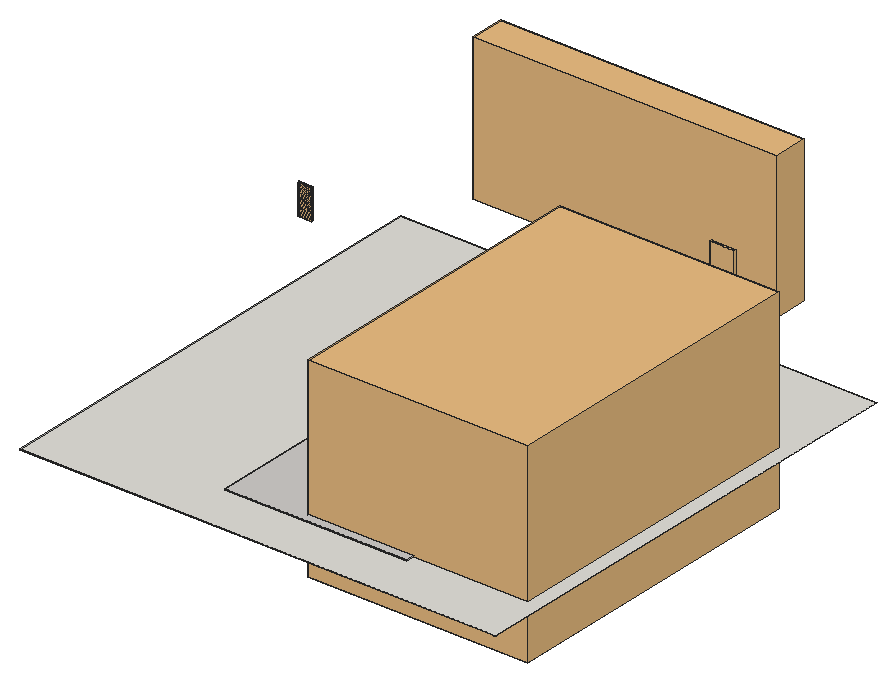
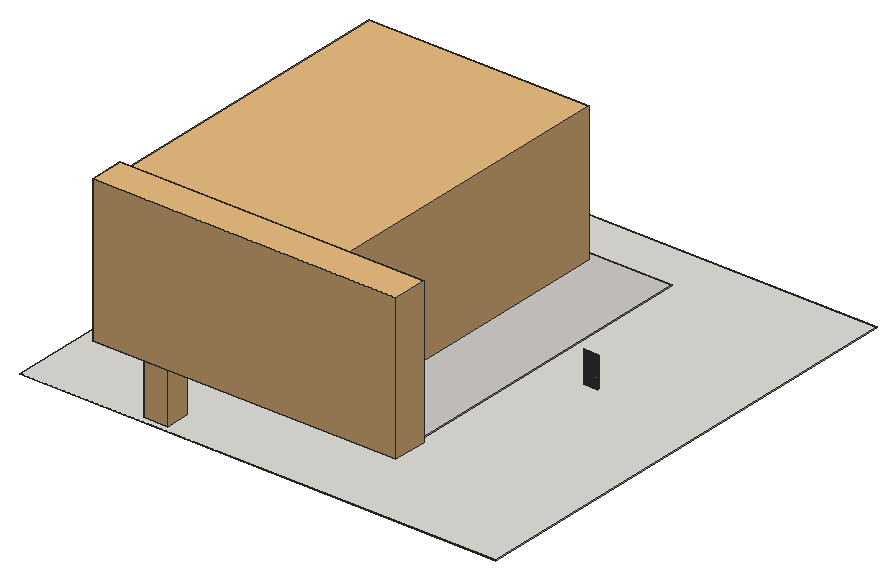
# SketchUp Ruby script. Lengths in inches.
U = 1.inch
M = Sketchup.active_model
def pt(a) = Geom::Point3d.new(a.map { |v| v * U })
def face(e, loops, mat)
  f = e.add_face(loops[0].map { |a| pt(a) })
  loops[1..].each { |l| e.add_face(l.map { |a| pt(a) }).erase! }
  f.material = f.back_material = mat if mat
  f
end
# faces: each face lists its corners as indices into pts; further lists are holes
def faces(e, pts, list, mat = nil) = list.each { |f| face(e, (f[0].is_a?(Array) ? f : [f]).map { |l| l.map { |i| pts[i] } }, mat) }
# xy, xz, yz: faces in a plane at the given z, y or x. An outline is a flat list of corners, or four numbers for a rectangle; further outlines are holes
def ring(l) = l.size == 4 ? [[l[0], l[1]], [l[2], l[1]], [l[2], l[3]], [l[0], l[3]]] : l.each_slice(2).to_a
def flat(e, list, mat, &to3) = list.each { |f| face(e, (f[0].is_a?(Array) ? f : [f]).map { |l| ring(l).map { |u, v| to3.(u, v) } }, mat) }
def xy(e, z, list, mat = nil) = flat(e, list, mat) { |x, y| [x, y, z] }
def xz(e, y, list, mat = nil) = flat(e, list, mat) { |x, z| [x, y, z] }
def yz(e, x, list, mat = nil) = flat(e, list, mat) { |y, z| [x, y, z] }
def lines(e, pts, list) = list.each { |a, b| e.add_line(pt(pts[a]), pt(pts[b])) }
# prism: a flat outline (further loops are holes) pulled along v
def prism(e, loops, v, mat = nil)
  f = face(e, loops, mat); d = Geom::Vector3d.new(v.map { |x| x * U })
  f.pushpull(f.normal.samedirection?(d) ? d.length : -d.length)
end
def box(e, o, s, mat = nil) = prism(e, [[o, [o[0] + s[0], o[1], o[2]], [o[0] + s[0], o[1] + s[1], o[2]], [o[0], o[1] + s[1], o[2]]]], [0, 0, s[2]], mat)
def at(x, y, z, deg = 0) = Geom::Transformation.translation(pt([x, y, z])) * Geom::Transformation.rotation(ORIGIN, Z_AXIS, deg.degrees)
def axes(o, x, y, z) = Geom::Transformation.new([*x, 0, *y, 0, *z, 0, *pt(o).to_a, 1])
def part(name) = M.definitions.add(name)
# library, detail: a bought-in or finely detailed component or shape, given as its bounding box
def library(name, o, s) = part(name).tap { |d| box(d.entities, o, s) }
def detail(e, o, s) = box(e.add_group.entities, o, s)
def put(e, d, t, mat = nil) = e.add_instance(d, t).tap { |i| i.material = mat if mat }
def group(e, t, mat = nil) = e.add_group.tap { |g| g.transformation = t; g.material = mat if mat }.entities
root = M.entities
M.materials.add("BED RUG").color = [207, 204, 201]
M.materials.add("[Marble Carrara Gold Floor Tile]").color = [225, 223, 217]
M.materials.add("green").color = [174, 139, 102]
c1 = part("3DGeom~106_Defintion")
p = [[13,-457.77,-202.36],[12.43,-457.8,-202.3125],[13.01,-486.125,-217.66],[13.55,-486.1,-217.7],[11.89,-399.92,-173.32],[11.84,-429.07,-187.52],
  [12.45,-429.04,-187.5625],[11.24,-399.94,-173.27],[10.74,-340.47,-146.51],[10.02,-340.5,-146.45],[10.64,-370.42,-159.59],[11.32,-370.39,-159.64],
  [9.74,-274.82,-123],[9.45,-308.6875,-134.19],[10.21,-308.66,-134.25],[8.94,-274.85,-122.9375],[8.71,-207.8125,-101.79],[7.83,-207.84,-101.72],
  [8.42,-240.67,-112.26],[9.26,-240.64,-112.32],[7.13,-153.09,-79.54],[7.1,-178.08,-90.92],[8.02,-178.05,-90.99],[6.18,-153.15,-79.48],
  [4,-118.48,-55.33],[4.82,-133.72,-67.51],[5.79,-133.63,-67.55],[3.02,-118.6,-55.3],[0.33,-95.6,-29.9375],[-0.7,-95.73,-29.92],
  [1.08,-106.39,-42.81],[2.09,-106.26,-42.82],[-1.44,-73.6,-2.8],[-2,-85.27,-16.55],[-0.96,-85.15,-16.59],[-2.51,-73.67,-2.71],
  [0.95,-49.78,26.84],[-1.83,-61.59,11.65],[-0.75,-61.55,11.52],[0.95,-49.78,26.84],[-0.16,-49.81,27.01],[5.32,-27.04,58.03],
  [2.02,-38.3,42.73],[3.14,-38.29,42.55],[5.32,-27.04,58.03],[4.18,-27.0625,58.2],[7.55,-5.16,85.82],[5.8,-16.06,72.8],
  [6.97,-16.01,72.65],[6.36,-5.25,85.91],[4.9,15.04,108.74],[3.7,14.85,108.73],[5.55,5,97.6],[6.74,5.15,97.57],
  [0,34.3,128.09],[-1.23,34.1,128.07],[1.28,24.49,118.99],[2.49,24.7,119.02],[-3.26,54.16,141.33],[-4.54,54.09,141.39],
  [-3.34,43.89,135.65],[-2.08,44.05,135.64],[1.2,113.2,138.8],[-0.38,104.875,137.27],[0.95,104.81,137.18],[-0.15,113.16,138.875],
  [0.07,95.73,138.14],[-2.47,86.16,140.63],[-1.16,86.02,140.55],[-1.25,95.85,138.22],[-2.41,75.83,143.01],[-3.7,75.9375,143.09],
  [-4.55,65.2,143.98],[-3.26,65.16,143.89],[-0.4,131.04,151.24],[-0.67,121.83,143.76],[0.69,121.94,143.73],[-1.77,130.9,151.24],
  [-3.3125,149.46,169.92],[-4.71,149.31,169.92],[-3.22,140.1,160.31],[-1.83,140.26,160.32],[-5.28,167.68,186.64],[-5.98,158.46,179.0625],
  [-4.5625,158.59,179.04],[-6.71,167.6,186.71],[-4.84,183.58,197.42],[-6.74,175.84,192.46],[-5.3,175.86,192.35],[-6.28,183.61,197.56],
  [-3.32,198.87,205.72],[-5.56,191.21,202.02],[-4.1,191.16,201.87],[-4.79,198.92,205.87],[-2.54,215.74,211.62],[-4.2,207,209.1],
  [-2.73,206.98,208.96],[-4.03,215.71,211.74],[-3.51,234.5625,213.875],[-4.36,225.09,213.4375],[-2.87,225.16,213.32],[-5.02,234.48,213.99],
  [-5.16,253.86,213.61],[-6.6875,253.77,213.74],[-5.84,243.98,213.93],[-4.32,244.07,213.8125],[-6.4,274.98,214.6],[-7.43,264.02,213.86],
  [-5.89,264.1,213.73],[-7.96,274.93,214.73],[-6.84,297.22,218.75],[-8.26,286.04,216.51],[-6.68,286.08,216.38],[-8.43,297.18,218.89],
  [-6.9375,322.55,224.28],[-8.52,309.11,221.61],[-6.91,309.14,221.48],[-8.56,322.52,224.42],[-6.99,356.56,229.06],[-8.59,338.11,227.04],
  [-6.95,338.125,226.9],[-8.65,356.54,229.2],[-7.09,400.64,232.43],[-8.73,377.54,230.99],[-7.05,377.56,230.84],[-8.81,400.63,232.57],
  [-7.16,453.07,235],[-8.875,425.8,233.96],[-7.13,425.81,233.8125],[-8.93,453.07,235.16],[-7.18,513.875,236.79],[-8.98,482.42,236.15],
  [-7.17,482.43,236],[-9.02,513.875,236.95]]
faces(c1.entities,p,[[0,1,2],[0,2,3],[4,5,6],[4,7,5],[8,9,10],[8,10,11],[12,13,14],[12,15,13],
  [16,17,18],[16,18,19],[20,21,22],[20,23,21],[24,25,26],[24,27,25],[28,29,30],[28,30,31],
  [32,33,34],[32,35,33],[36,37,38],[39,40,37],[41,42,43],[44,45,42],[46,47,48],[46,49,47],
  [50,51,52],[50,52,53],[54,55,56],[54,56,57],[58,59,60],[58,60,61],[62,63,64],[62,65,63],
  [66,67,68],[66,69,67],[70,71,72],[70,72,73],[74,75,76],[74,77,75],[78,79,80],[78,80,81],
  [82,83,84],[82,85,83],[86,87,88],[86,89,87],[90,91,92],[90,93,91],[94,95,96],[94,97,95],
  [98,99,100],[98,101,99],[102,103,104],[102,104,105],[106,107,108],[106,109,107],[110,111,112],[110,113,111],
  [114,115,116],[114,117,115],[118,119,120],[118,121,119],[122,123,124],[122,125,123],[126,127,128],[126,129,127],
  [130,131,132],[130,133,131]],"green")
c2 = part("3DGeom~107_Defintion")
p = [[13.6,-487.82,-218.47],[13.05,-487.84,-218.43],[13.63,-515.87,-234.39],[14.13,-515.85,-234.43],[12.5,-430.56,-188.23],[12.47,-459.41,-203.03],
  [13.05,-459.39,-203.07],[11.88,-430.58,-188.18],[11.36,-371.7,-160.2],[10.67,-371.73,-160.15],[11.28,-401.36,-173.89],[11.93,-401.33,-173.94],
  [10.25,-309.75,-134.72],[9.49,-309.78,-134.66],[10.06,-341.7,-146.97],[10.78,-341.67,-147.02],[9.29,-241.49,-112.72],[8.45,-241.52,-112.65],
  [8.97,-275.82,-123.37],[9.77,-275.8,-123.4375],[8.05,-178.67,-91.3125],[7.86,-208.57,-102.08],[8.74,-208.55,-102.15],[7.13,-178.71,-91.24],
  [5.81,-134.1,-67.79],[4.83,-134.1875,-67.74],[6.2,-153.69,-79.76],[7.16,-153.63,-79.82],[2.09,-106.64,-42.97],[1.09,-106.77,-42.96],
  [3.03,-119.01,-55.5],[4.02,-118.9,-55.53],[-0.96,-85.46,-16.65],[-2.01,-85.57,-16.6],[-0.7,-96.07,-30.02],[0.33,-95.9375,-30.04],
  [-0.75,-61.77,11.56],[-2.52,-73.93,-2.72],[-1.45,-73.86,-2.81],[-1.84,-61.81,11.7],[3.15,-38.42,42.7],[-0.16,-49.98,27.1],
  [0.95,-49.96,26.9375],[2.03,-38.4375,42.88],[6.99,-16.07,72.91],[4.19,-27.16,58.41],[5.34,-27.14,58.23],[5.82,-16.12,73.06],
  [6.77,5.17,97.91],[6.39,-5.26,86.21],[7.58,-5.17,86.12],[5.56,5.02,97.95],[2.5,24.78,119.4375],[1.28,24.58,119.41],
  [3.71,14.9,109.11],[4.92,15.09,109.12],[-2.09,44.21,136.12],[-3.35,44.05,136.13],[-1.23,34.22,128.52],[0,34.42,128.54],
  [0.96,105.18,137.67],[-1.25,96.19,138.71],[0.07,96.06,138.625],[-0.38,105.24,137.76],[0.7,122.37,144.24],[-0.15,113.56,139.37],
  [1.21,113.6,139.29],[-0.67,122.26,144.27],[-1.17,86.33,141.05],[-3.72,76.2,143.59],[-2.41,76.09,143.51],[-2.48,86.46,141.125],
  [-3.27,65.39,144.4],[-4.56,54.28,141.89],[-3.27,54.35,141.83],[-4.57,65.43,144.49],[-1.84,140.75,160.88],[-3.23,140.59,160.875],
  [-1.78,131.36,151.78],[-0.41,131.5,151.77],[-4.58,159.15,179.67],[-6,159.02,179.69],[-4.73,149.83,170.52],[-3.33,149.99,170.52],
  [-5.32,176.48,193.03],[-6.74,168.19,187.37],[-5.3,168.27,187.3],[-6.76,176.46,193.14],[-4.12,191.83,202.58],[-6.31,184.26,198.26],
  [-4.85,184.23,198.12],[-5.58,191.88,202.74],[-2.73,207.71,209.7],[-4.8,199.62,206.59],[-3.33,199.57,206.44],[-4.22,207.73,209.84],
  [-2.875,225.96,214.07],[-4.05,216.47,212.49],[-2.55,216.5,212.36],[-4.38,225.89,214.19],[-5.91,265.03,214.49],[-6.71,254.67,214.49],
  [-5.17,254.76,214.37],[-7.46,264.96,214.61],[-4.33,244.9375,214.57],[-5.86,244.84,214.6875],[-5.03,235.3,214.75],[-3.52,235.39,214.63],
  [-6.71,287.09,217.15],[-7.99,275.9,215.49],[-6.42,275.95,215.36],[-8.29,287.05,217.28],[-6.9375,310.23,222.26],[-8.46,298.23,219.66],
  [-6.87,298.27,219.53],[-8.55,310.2,222.39],[-6.97,339.32,227.7],[-8.59,323.66,225.21],[-6.96,323.68,225.07],[-8.62,339.3,227.84],
  [-7.07,378.89,231.66],[-8.68,357.8,230.01],[-7.02,357.82,229.87],[-8.76,378.88,231.8],[-7.16,427.3125,234.64],[-8.84,402.04,233.39],
  [-7.12,402.05,233.25],[-8.91,427.31,234.79],[-7.2,484.13,236.83],[-8.96,454.67,235.99],[-7.18,454.67,235.83],[-9.01,484.125,236.99]]
faces(c2.entities,p,[[0,1,2],[0,2,3],[4,5,6],[4,7,5],[8,9,10],[8,10,11],[12,13,14],[12,14,15],
  [16,17,18],[16,18,19],[20,21,22],[20,23,21],[24,25,26],[24,26,27],[28,29,30],[28,30,31],
  [32,33,34],[32,34,35],[36,37,38],[36,39,37],[40,41,42],[40,43,41],[44,45,46],[44,47,45],
  [48,49,50],[48,51,49],[52,53,54],[52,54,55],[56,57,58],[56,58,59],[60,61,62],[60,63,61],
  [64,65,66],[64,67,65],[68,69,70],[68,71,69],[72,73,74],[72,75,73],[76,77,78],[76,78,79],
  [80,81,82],[80,82,83],[84,85,86],[84,87,85],[88,89,90],[88,91,89],[92,93,94],[92,95,93],
  [96,97,98],[96,99,97],[100,101,102],[100,103,101],[104,105,106],[104,106,107],[108,109,110],[108,111,109],
  [112,113,114],[112,115,113],[116,117,118],[116,119,117],[120,121,122],[120,123,121],[124,125,126],[124,127,125],
  [128,129,130],[128,131,129]],"green")
c3 = library("3DGeom~108_Defintion",[-15.55,-485.98,-221.31],[30.67,1000,457.14])
c4 = library("3DGeom~109_Defintion",[-10.83,-486.12,-217.86],[24.87,1000,454.81])
c5 = library("3DGeom~110_Defintion",[-15.46,-515.69,-237.75],[31.06,1000,473.61])
c6 = library("3DGeom~111_Defintion",[-10.8,-515.86,-234.58],[25.39,1000,471.56])
c7 = library("3DGeom~112_Defintion",[-15.55,-486.02,-221.29],[30.67,1000,457.87])
c8 = library("3DGeom~113_Defintion",[-15.46,-515.73,-237.74],[31.06,1000,474.35])
c9 = part("3DGeom~114_Defintion")
p = [[13.375,-498.625,-230.47],[14.29,-498.73,-230.21],[11.9375,-499.79,-227.73],[12.4375,-498.72,-230.29],[13.375,-498.625,-230.47],[11.9375,-499.79,-227.73],
  [12.4375,-498.72,-230.29],[12.89,-498.65,-230.4375],[13.375,-498.625,-230.47],[13.375,-498.625,-230.47],[13.86,-498.65,-230.39],[14.29,-498.73,-230.21],
  [11.67,-499.65,-228.07],[12.4375,-498.72,-230.29],[11.9375,-499.79,-227.73],[11.67,-499.65,-228.07],[12.06,-498.82,-230.05],[12.4375,-498.72,-230.29],
  [14.29,-498.73,-230.21],[14.92,-498.98,-229.58],[11.9375,-499.79,-227.73],[14.29,-498.73,-230.21],[14.65,-498.83,-229.93],[14.92,-498.98,-229.58],
  [11.5,-499.49,-228.48],[12.06,-498.82,-230.05],[11.67,-499.65,-228.07],[11.5,-499.49,-228.48],[11.75,-498.96,-229.73],[12.06,-498.82,-230.05],
  [11.75,-498.96,-229.73],[11.5,-499.49,-228.48],[11.46,-499.3,-228.92],[11.75,-498.96,-229.73],[11.46,-499.3,-228.92],[11.55,-499.12,-229.35],
  [14.92,-498.98,-229.58],[15.125,-499.32,-228.74],[11.9375,-499.79,-227.73],[14.92,-498.98,-229.58],[15.08,-499.14,-229.18],[15.125,-499.32,-228.74],
  [15.125,-499.32,-228.74],[14.83,-499.67,-227.92],[11.9375,-499.79,-227.73],[15.125,-499.32,-228.74],[15.04,-499.51,-228.31],[14.83,-499.67,-227.92],
  [14.83,-499.67,-227.92],[14.15,-499.91,-227.36],[11.9375,-499.79,-227.73],[14.83,-499.67,-227.92],[14.53,-499.81,-227.6],[14.15,-499.91,-227.36],
  [13.21,-500,-227.18],[12.3,-499.9,-227.45],[11.9375,-499.79,-227.73],[14.15,-499.91,-227.36],[13.21,-500,-227.18],[11.9375,-499.79,-227.73],
  [13.21,-500,-227.18],[12.73,-499.97,-227.27],[12.3,-499.9,-227.45],[14.15,-499.91,-227.36],[13.7,-499.98,-227.22],[13.21,-500,-227.18],
  [-8.13,500,217.125],[-13.4,499.85,228.29],[-4.81,499.99,218.2],[-11.54,499.99,217.875],[-13.4,499.85,228.29],[-8.13,500,217.125],
  [-11.54,499.99,217.875],[-8.13,500,217.125],[-9.91,500,217.28],[-8.13,500,217.125],[-4.81,499.99,218.2],[-6.37,500,217.45],
  [-14.375,499.87,226.89],[-13.4,499.85,228.29],[-11.54,499.99,217.875],[-14.375,499.87,226.89],[-11.54,499.99,217.875],[-12.94,499.97,218.85],
  [-4.81,499.99,218.2],[-13.4,499.85,228.29],[-2.53,499.96,220.71],[-4.81,499.99,218.2],[-2.53,499.96,220.71],[-3.5,499.97,219.31],
  [-14.97,499.89,225.26],[-14.375,499.87,226.89],[-12.94,499.97,218.85],[-14.97,499.89,225.26],[-12.94,499.97,218.85],[-14.05,499.96,220.15],
  [-15.125,499.91,223.48],[-14.97,499.89,225.26],[-14.05,499.96,220.15],[-15.125,499.91,223.48],[-14.05,499.96,220.15],[-14.8,499.9375,221.72],
  [-2.53,499.96,220.71],[-13.4,499.85,228.29],[-1.77,499.91,224.12],[-2.53,499.96,220.71],[-1.77,499.91,224.12],[-1.93,499.9375,222.34],
  [-1.77,499.91,224.12],[-13.4,499.85,228.29],[-2.85,499.87,227.44],[-1.77,499.91,224.12],[-2.85,499.87,227.44],[-2.1,499.89,225.88],
  [-2.85,499.87,227.44],[-13.4,499.85,228.29],[-5.36,499.84,229.72],[-2.85,499.87,227.44],[-5.36,499.84,229.72],[-3.96,499.85,228.74],
  [-8.77,499.83,230.47],[-13.4,499.85,228.29],[-12.09,499.84,229.4],[-5.36,499.84,229.72],[-13.4,499.85,228.29],[-8.77,499.83,230.47],
  [-8.77,499.83,230.47],[-12.09,499.84,229.4],[-10.53,499.83,230.15],[-5.36,499.84,229.72],[-8.77,499.83,230.47],[-6.99,499.83,230.32]]
faces(c9.entities,p,[[0,1,2],[3,4,5],[6,7,8],[9,10,11],[12,13,14],[15,16,17],[18,19,20],[21,22,23],
  [24,25,26],[27,28,29],[30,31,32],[33,34,35],[36,37,38],[39,40,41],[42,43,44],[45,46,47],
  [48,49,50],[51,52,53],[54,55,56],[57,58,59],[60,61,62],[63,64,65],[66,67,68],[69,70,71],
  [72,73,74],[75,76,77],[78,79,80],[81,82,83],[84,85,86],[87,88,89],[90,91,92],[93,94,95],
  [96,97,98],[99,100,101],[102,103,104],[105,106,107],[108,109,110],[111,112,113],[114,115,116],[117,118,119],
  [120,121,122],[123,124,125],[126,127,128],[129,130,131]],"green")
c10 = library("Shelve 2",[0,0,0],[15.49,139.2,58.51])
c11 = part("Area rug")
box(c11.entities,[0,0,0],[60,96,0.5],"BED RUG")
c12 = part("BED RUG")
put(c12.entities,c11,at(0,0,0))
c13 = library("STANDLAMP CYLINDER SHADE",[-20.4,-20.4,-130.73],[40.8,40.8,185.38])
c14 = library("Sectional sofa",[-0.93,-10.63,-23.92],[126.92,88.46,78.25])
g1 = group(root,at(15.3125,134.49,26.21))
put(g1,c1,axes([2.7,0.5625,11.18],[0,0.01211,0],[0,0,-0.01211],[-0.01211,0,0]),"green")
put(g1,c2,axes([2.7,0.5625,11.18],[0,0.01207,0],[0,0,-0.01207],[-0.01207,0,0]),"green")
put(g1,c3,axes([2.7,0.5625,11.18],[0,0.01211,0],[0,0,-0.01211],[-0.01211,0,0]),"green")
put(g1,c4,axes([2.7,0.5625,11.18],[0,0.01211,0],[0,0,-0.01211],[-0.01211,0,0]),"green")
put(g1,c5,axes([2.7,0.5625,11.18],[0,0.01207,0],[0,0,-0.01207],[-0.01207,0,0]),"green")
put(g1,c6,axes([2.7,0.5625,11.18],[0,0.01207,0],[0,0,-0.01207],[-0.01207,0,0]),"green")
put(g1,c7,axes([2.7,0.5625,11.18],[0,0.01211,0],[0,0,-0.01211],[-0.01211,0,0]),"green")
put(g1,c8,axes([2.7,0.5625,11.18],[0,0.01207,0],[0,0,-0.01207],[-0.01207,0,0]),"green")
put(g1,c9,axes([2.7,0.5625,11.18],[0,0.01245,0],[0,0,-0.01245],[-0.01245,0,0]),"green")
g2 = group(root,at(198,6,0,90))
xy(g2,0,[[0,0,192,192]])
xy(g2,0.25,[[0,0,192,192]],"[Marble Carrara Gold Floor Tile]")
xz(g2,0,[[0,0,192,0.25]])
xz(g2,192,[[0,0,192,0.25]])
yz(g2,0,[[0,0,192,0.25]])
yz(g2,192,[[0,0,192,0.25]])
put(root,c10,axes([44.04,200.9375,24.62],[0,-0.9,0],[0.88,0,0],[0,0,1]))
put(root,c12,axes([146,154.91,0.25],[-1.22,0,0],[0,-1.3447,0],[0,0,1]))
put(root,c13,axes([145.29,190.83,30.84],[0,0.234,0],[-0.234,0,0],[0,0,0.234]))
put(root,c14,at(181.32,30.39,1.99,90))
